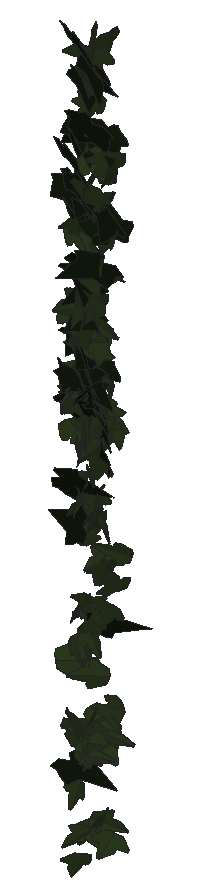
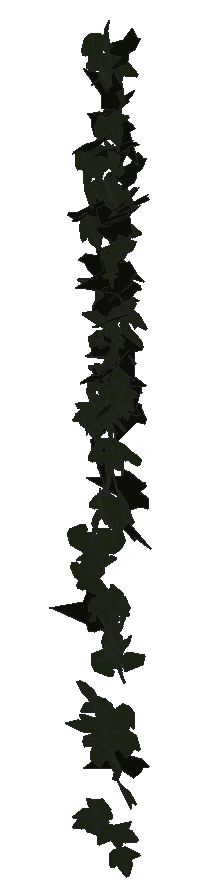
# SketchUp Ruby script. Lengths in inches.
U = 1.inch
M = Sketchup.active_model
def pt(a) = Geom::Point3d.new(a.map { |v| v * U })
def face(e, loops, mat)
  f = e.add_face(loops[0].map { |a| pt(a) })
  loops[1..].each { |l| e.add_face(l.map { |a| pt(a) }).erase! }
  f.material = f.back_material = mat if mat
  f
end
# faces: each face lists its corners as indices into pts; further lists are holes
def faces(e, pts, list, mat = nil) = list.each { |f| face(e, (f[0].is_a?(Array) ? f : [f]).map { |l| l.map { |i| pts[i] } }, mat) }
# xy, xz, yz: faces in a plane at the given z, y or x. An outline is a flat list of corners, or four numbers for a rectangle; further outlines are holes
def ring(l) = l.size == 4 ? [[l[0], l[1]], [l[2], l[1]], [l[2], l[3]], [l[0], l[3]]] : l.each_slice(2).to_a
def flat(e, list, mat, &to3) = list.each { |f| face(e, (f[0].is_a?(Array) ? f : [f]).map { |l| ring(l).map { |u, v| to3.(u, v) } }, mat) }
def xy(e, z, list, mat = nil) = flat(e, list, mat) { |x, y| [x, y, z] }
def xz(e, y, list, mat = nil) = flat(e, list, mat) { |x, z| [x, y, z] }
def yz(e, x, list, mat = nil) = flat(e, list, mat) { |y, z| [x, y, z] }
def lines(e, pts, list) = list.each { |a, b| e.add_line(pt(pts[a]), pt(pts[b])) }
# prism: a flat outline (further loops are holes) pulled along v
def prism(e, loops, v, mat = nil)
  f = face(e, loops, mat); d = Geom::Vector3d.new(v.map { |x| x * U })
  f.pushpull(f.normal.samedirection?(d) ? d.length : -d.length)
end
def box(e, o, s, mat = nil) = prism(e, [[o, [o[0] + s[0], o[1], o[2]], [o[0] + s[0], o[1] + s[1], o[2]], [o[0], o[1] + s[1], o[2]]]], [0, 0, s[2]], mat)
def at(x, y, z, deg = 0) = Geom::Transformation.translation(pt([x, y, z])) * Geom::Transformation.rotation(ORIGIN, Z_AXIS, deg.degrees)
def axes(o, x, y, z) = Geom::Transformation.new([*x, 0, *y, 0, *z, 0, *pt(o).to_a, 1])
def part(name) = M.definitions.add(name)
# library, detail: a bought-in or finely detailed component or shape, given as its bounding box
def library(name, o, s) = part(name).tap { |d| box(d.entities, o, s) }
def detail(e, o, s) = box(e.add_group.entities, o, s)
def put(e, d, t, mat = nil) = e.add_instance(d, t).tap { |i| i.material = mat if mat }
def group(e, t, mat = nil) = e.add_group.tap { |g| g.transformation = t; g.material = mat if mat }.entities
root = M.entities
M.materials.add("1026 AP 7946 SUNNY SIDE UP").color = [254, 231, 186]
M.materials.add("efeu1").color = [18, 25, 13]
M.materials.add("efeu2").color = [43, 57, 29]
c1 = part("ivyleaf_9")
p = [[1.54,2.16,1.25],[1.36,2.04,1.19],[-0.21,0.99,0.68],[-0.71,1.11,0.82],[-0.85,0.86,0.67],[-0.8,0.17,0.21],
  [-0.9,-0.01,0.1],[-0.67,-0.16,-0.02],[-0.08,-0.08,-0.05],[-0.03,-0.6,-0.4],[0.65,-0.88,-0.66],[0.83,-0.6,-0.49],
  [1.29,-0.42,-0.43],[1.8125,-0.07,-0.26],[1.21,0.44,0.15]]
faces(c1.entities,p,[[0,1,2,3,4,5,6,7,8,9,10,11,12,13,14]],"efeu1")
c2 = part("ivyleaf_10")
p = [[0,0.5,-0.03],[-0.0625,2.02,-0.43],[-0.19,2.01,-0.46],[-0.54,1.05,-0.29],[-0.52,0.625,-0.18],[-0.83,0.76,-0.28],
  [-1.16,0.64,-0.33],[-1.15,0.33,-0.24],[-0.77,-0.39,0.02],[-0.3,-0.51,0.16],[0.04,-0.48,0.23],[-0.02,2.01,-0.4375],
  [-0.06,2.01,-0.43],[0.04,-0.49,0.23],[0.67,-0.49,0.14],[1.38,0.36,-0.2],[1.375,0.51,-0.24],[0.81,0.65,-0.19],
  [0.62,0.59,-0.15],[0.6,1.09,-0.28],[0.5,1.23,-0.31]]
faces(c2.entities,p,[[0,1,2,3,4,5,6,7,8,9,10],[11,12,0,13,14,15,16,17,18,19,20]],"efeu2")
put(root,c1,axes([104.4,212.4,264.42],[0.02989,-0.26168,-0.05002],[-0.00858,0.0468,-0.27001],[0.41798,0.01967,-0.00197]),"1026 AP 7946 SUNNY SIDE UP")
put(root,c1,axes([104.31,212.37,265.12],[0.20144,-0.21294,0.07682],[0.04069,-0.07271,-0.25599],[0.35306,0.12988,-0.01432]),"1026 AP 7946 SUNNY SIDE UP")
put(root,c2,axes([104.32,212.5625,259.23],[0.25489,0.03596,0.15428],[0.23922,-0.00544,-0.16856],[-0.03566,0.22049,-0.028]),"1026 AP 7946 SUNNY SIDE UP")
put(root,c1,axes([104.85,212.17,257.49],[-0.16935,-0.01867,-0.23851],[-0.36458,0.02183,0.10948],[0.01886,0.25432,-0.0254]),"1026 AP 7946 SUNNY SIDE UP")
put(root,c2,axes([104.61,212.53,260.5],[0.32823,-0.01925,-0.08265],[-0.12677,-0.00257,-0.21576],[0.02681,0.22358,-0.00828]),"1026 AP 7946 SUNNY SIDE UP")
put(root,c2,axes([104.83,212.23,262.04],[-0.19983,0.01215,0.215],[-0.3172,-0.0709,-0.12276],[0.08582,-0.23378,0.04691]),"1026 AP 7946 SUNNY SIDE UP")
put(root,c2,axes([104.5,212.45,253.1],[-0.29451,-0.02372,-0.08377],[0.13034,-0.01233,-0.19339],[0.02639,-0.20377,0.02024]),"1026 AP 7946 SUNNY SIDE UP")
put(root,c2,axes([104.37,212.42,261.75],[0.28025,-0.04811,0.18082],[0.24774,-0.08293,-0.18843],[0.14407,0.2362,-0.02772]),"1026 AP 7946 SUNNY SIDE UP")
put(root,c1,axes([104.74,212.24,260.06],[0.1133,-0.04955,0.23654],[-0.1924,0.19742,0.08451],[-0.31578,-0.13807,0.03338]),"1026 AP 7946 SUNNY SIDE UP")
put(root,c1,axes([104.5,212.41,265.51],[0.24093,-0.15823,-0.14785],[-0.17433,0.09078,-0.22593],[0.28602,0.18862,-0.01316]),"1026 AP 7946 SUNNY SIDE UP")
put(root,c2,axes([104.59,212.35,260.125],[0.03534,-0.14597,0.17818],[0.046,-0.17132,-0.15314],[0.35389,0.03684,0.00211]),"1026 AP 7946 SUNNY SIDE UP")
put(root,c2,axes([104.6,212.45,257.78],[-0.07078,-0.19746,-0.10932],[0.05848,0.099,-0.20766],[0.34676,-0.057,0.01271]),"1026 AP 7946 SUNNY SIDE UP")
put(root,c2,axes([104.65,212.36,263.78],[-0.11542,-0.23449,-0.01715],[0.00878,0.0143,-0.25304],[0.36939,-0.07361,0.00066]),"1026 AP 7946 SUNNY SIDE UP")
put(root,c1,axes([104.53,212.66,264.17],[-0.11975,-0.19196,0.15357],[0.03496,-0.16214,-0.20286],[0.38162,-0.04539,0.06677]),"1026 AP 7946 SUNNY SIDE UP")
put(root,c2,axes([104.6875,212.45,257.67],[-0.22727,0.15109,-0.03318],[-0.02909,0.02804,0.21548],[0.24145,0.14559,-0.00527]),"1026 AP 7946 SUNNY SIDE UP")
put(root,c1,axes([104.44,212.47,264.52],[0.14828,-0.23824,0.00096],[-0.0061,-0.00399,-0.26393],[0.37458,0.09425,-0.00468]),"1026 AP 7946 SUNNY SIDE UP")
put(root,c2,axes([104.53,212.4,263.51],[0.11016,0.22946,0.07194],[0.04535,0.0628,-0.24662],[-0.37381,0.07524,-0.00872]),"1026 AP 7946 SUNNY SIDE UP")
put(root,c1,axes([104.61,212.23,260],[0.33334,0.0588,-0.11051],[-0.15105,-0.05394,-0.22564],[-0.11984,0.23154,-0.02299]),"1026 AP 7946 SUNNY SIDE UP")
put(root,c2,axes([104.7,212.26,258.9],[0.00661,-0.00651,-0.23275],[-0.03665,0.22472,-0.00581],[0.35345,0.02342,0.00375]),"1026 AP 7946 SUNNY SIDE UP")
put(root,c2,axes([104.65,212.47,252.3125],[0.13679,-0.14464,0.12123],[-0.08114,0.10705,0.17426],[-0.28259,-0.10075,0.00865]),"1026 AP 7946 SUNNY SIDE UP")
put(root,c1,axes([104.76,212.44,261.4],[0.14498,0.12771,-0.19277],[-0.14162,-0.16555,-0.16247],[-0.32788,0.12798,-0.01506]),"1026 AP 7946 SUNNY SIDE UP")
put(root,c2,axes([104.64,212.17,253.39],[-0.25694,0.13165,-0.01009],[-0.00282,-0.01898,-0.21567],[-0.20765,-0.16264,0.01542]),"1026 AP 7946 SUNNY SIDE UP")
put(root,c2,axes([104.73,212.35,260.19],[-0.18599,-0.15209,0.15492],[-0.05259,-0.15753,-0.19106],[0.33314,-0.10978,0.05633]),"1026 AP 7946 SUNNY SIDE UP")
put(root,c2,axes([104.61,212.34,251.87],[0.27254,-0.13581,0.04207],[0.0368,-0.03744,-0.22655],[0.22029,0.17427,-0.01421]),"1026 AP 7946 SUNNY SIDE UP")
put(root,c2,axes([104.71,212.39,250.9],[-0.04074,-0.1,0.1821],[-0.03764,-0.17602,-0.10689],[0.31789,-0.03365,0.01068]),"1026 AP 7946 SUNNY SIDE UP")
put(root,c2,axes([104.82,212.09,262.1],[0.08822,-0.12808,-0.23163],[-0.19621,0.18731,-0.14137],[0.35531,0.13524,-0.02056]),"1026 AP 7946 SUNNY SIDE UP")
put(root,c2,axes([104.71,212.3125,250.41],[-0.13218,-0.17999,0.05105],[-0.01944,-0.04998,-0.20471],[0.29334,-0.08442,0.00944]),"1026 AP 7946 SUNNY SIDE UP")
put(root,c2,axes([104.64,212.59,259.1],[0.2023,0.1578,-0.05612],[-0.03973,-0.05072,-0.20968],[-0.25994,0.13056,-0.01163]),"1026 AP 7946 SUNNY SIDE UP")
put(root,c1,axes([104.34,212.26,258.27],[0.17162,0.03856,-0.22421],[0.27273,0.13589,0.11509],[0.21596,-0.20225,0.03282]),"1026 AP 7946 SUNNY SIDE UP")
put(root,c2,axes([104.73,212.48,266.17],[0.22106,-0.17971,-0.14914],[-0.0654,0.14583,-0.22888],[0.3559,0.13842,0.05058]),"1026 AP 7946 SUNNY SIDE UP")
put(root,c2,axes([104.72,212.44,254.66],[0.16577,-0.18209,-0.04436],[-0.0454,0.0318,-0.21638],[0.29032,0.10895,-0.00851]),"1026 AP 7946 SUNNY SIDE UP")
put(root,c1,axes([104.52,212.35,264.1],[0.20084,-0.20444,-0.05932],[-0.04789,0.0475,-0.24806],[0.33002,0.13131,0.00011]),"1026 AP 7946 SUNNY SIDE UP")
put(root,c2,axes([104.64,212.38,261.36],[-0.03415,-0.13729,-0.19819],[0.11714,0.17855,-0.13945],[0.35163,-0.07281,0.02721]),"1026 AP 7946 SUNNY SIDE UP")
put(root,c2,axes([104.64,212.27,254.9375],[0.02045,0.21136,0.01667],[0.00065,0.01498,-0.21806],[-0.33317,0.013,0.0006]),"1026 AP 7946 SUNNY SIDE UP")
put(root,c2,axes([104.72,212.21,255.74],[0.05952,-0.17736,-0.11889],[0.00236,0.11645,-0.18479],[0.33185,0.03099,0.02264]),"1026 AP 7946 SUNNY SIDE UP")
put(root,c2,axes([104.72,212.56,255.27],[0.05189,-0.21191,0.05899],[0.00316,-0.05882,-0.22117],[0.34564,0.03235,-0.00684]),"1026 AP 7946 SUNNY SIDE UP")
put(root,c2,axes([104.625,212.47,265.23],[0.18103,-0.23237,0.04226],[0.01082,0.05038,0.26587],[-0.37123,-0.11185,0.02836]),"1026 AP 7946 SUNNY SIDE UP")
put(root,c2,axes([104.48,212.13,254.57],[0.09186,-0.06714,-0.2225],[0.30328,0.13064,0.01269],[0.18463,-0.18119,0.08985]),"1026 AP 7946 SUNNY SIDE UP")
put(root,c2,axes([104.77,212.25,260.29],[-0.32411,0.15872,-0.0115],[0.00397,0.023,0.26737],[0.25027,0.20519,-0.01914]),"1026 AP 7946 SUNNY SIDE UP")
put(root,c2,axes([104.77,212.65,266.16],[-0.13137,-0.20015,0.13279],[0.00083,-0.13793,-0.21916],[0.3753,-0.06975,0.04697]),"1026 AP 7946 SUNNY SIDE UP")
put(root,c2,axes([104.63,212.46,258.29],[0.23018,-0.13321,0.11784],[0.12203,-0.08559,-0.20416],[0.24851,0.16541,-0.00889]),"1026 AP 7946 SUNNY SIDE UP")
put(root,c1,axes([104.72,212.36,261.11],[0.20799,-0.09581,-0.19009],[-0.24572,0.09747,-0.16746],[0.21449,0.20456,-0.00751]),"1026 AP 7946 SUNNY SIDE UP")
put(root,c1,axes([104.63,212.58,265.63],[-0.07708,-0.24624,-0.01975],[0.01844,0.01578,-0.25842],[0.38776,-0.0497,0.00836]),"1026 AP 7946 SUNNY SIDE UP")
put(root,c1,axes([104.58,212.625,266.51],[-0.02104,-0.2071,0.15439],[0.05871,-0.15121,-0.21107],[0.39875,0.01134,0.03922]),"1026 AP 7946 SUNNY SIDE UP")
put(root,c2,axes([104.53,212.41,252.93],[-0.12964,-0.0363,-0.1905],[0.29283,0.01369,-0.08833],[0.04318,-0.20182,0.02705]),"1026 AP 7946 SUNNY SIDE UP")
put(root,c1,axes([104.5,212.67,263.93],[-0.03753,-0.05014,0.24504],[0.24353,-0.1877,-0.02582],[0.29517,0.14849,0.05246]),"1026 AP 7946 SUNNY SIDE UP")
put(root,c1,axes([104.62,212.47,262.51],[-0.00964,-0.20211,0.13903],[0.02701,-0.13616,-0.2083],[0.38218,0.00452,0.01823]),"1026 AP 7946 SUNNY SIDE UP")
put(root,c2,axes([104.74,212.38,260.66],[-0.21966,0.20066,-0.01863],[-0.00032,-0.02353,-0.25163],[-0.31697,-0.13904,0.01316]),"1026 AP 7946 SUNNY SIDE UP")
put(root,c1,axes([104.49,212.37,262.78],[0.31408,0.07032,0.15021],[0.23278,0.01278,-0.21579],[-0.10157,0.24674,-0.03007]),"1026 AP 7946 SUNNY SIDE UP")
put(root,c1,axes([104.71,212.55,260.96],[-0.09346,-0.15157,0.20757],[-0.03004,-0.20458,-0.16485],[0.3964,-0.05124,0.03645]),"1026 AP 7946 SUNNY SIDE UP")
put(root,c2,axes([104.77,212.51,255.58],[-0.23717,0.14431,-0.00769],[-0.00694,-0.01657,-0.21459],[-0.22719,-0.15015,0.01459]),"1026 AP 7946 SUNNY SIDE UP")
put(root,c1,axes([104.83,212.59,262.38],[-0.02623,-0.04337,-0.24879],[0.10637,-0.23324,0.03701],[-0.37046,-0.0639,0.02824]),"1026 AP 7946 SUNNY SIDE UP")
put(root,c1,axes([104.53,212.33,267.59],[0.18723,-0.21887,0.12623],[0.08053,-0.11296,-0.25721],[0.38707,0.12937,-0.00754]),"1026 AP 7946 SUNNY SIDE UP")
put(root,c2,axes([104.66,212.25,260.01],[-0.22955,-0.1153,-0.16355],[0.23175,0.06496,-0.18863],[0.20239,-0.20515,0.03049]),"1026 AP 7946 SUNNY SIDE UP")
put(root,c2,axes([104.88,212.49,255.76],[-0.34473,-0.03433,0.04347],[-0.05951,-0.03074,-0.22744],[0.06178,-0.22117,0.02351]),"1026 AP 7946 SUNNY SIDE UP")
put(root,c2,axes([104.85,212.43,267.32],[-0.39172,-0.10153,0.00081],[0.01231,-0.02279,-0.27616],[0.15919,-0.24808,0.02334]),"1026 AP 7946 SUNNY SIDE UP")
put(root,c2,axes([104.84,212.5,257.98],[-0.29732,-0.09767,-0.00009],[0.01236,-0.01623,-0.21855],[0.15308,-0.18839,0.01747]),"1026 AP 7946 SUNNY SIDE UP")
put(root,c2,axes([104.98,212.26,262.22],[-0.32027,-0.04262,0.12058],[-0.1683,-0.05578,-0.21269],[0.1009,-0.22832,0.02799]),"1026 AP 7946 SUNNY SIDE UP")
put(root,c2,axes([105.05,212.38,261.32],[0.21917,-0.05349,-0.22711],[-0.33627,0.05428,-0.15275],[0.11761,0.25485,-0.01351]),"1026 AP 7946 SUNNY SIDE UP")
put(root,c1,axes([104.87,212.52,261.81],[-0.22125,-0.14511,0.15397],[-0.08418,-0.15009,-0.20182],[0.31751,-0.14091,0.05378]),"1026 AP 7946 SUNNY SIDE UP")
put(root,c2,axes([104.75,212.39,257.07],[-0.00794,-0.18001,0.14148],[0.03375,0.13739,0.18577],[-0.3554,0.01707,0.01448]),"1026 AP 7946 SUNNY SIDE UP")
put(root,c1,axes([105.03,212.23,265.94],[0.15446,0.02989,-0.25704],[-0.34671,-0.11861,-0.10469],[-0.19006,0.24066,-0.01791]),"1026 AP 7946 SUNNY SIDE UP")
put(root,c2,axes([104.86,212.27,261.94],[0.10784,-0.19761,-0.12152],[0.00674,0.12302,-0.21104],[0.3609,0.05675,0.04026]),"1026 AP 7946 SUNNY SIDE UP")
put(root,c2,axes([104.58,212.52,266.59],[-0.10393,0.03422,0.2773],[0.37706,-0.12185,0.07596],[0.199,0.24874,0.00089]),"1026 AP 7946 SUNNY SIDE UP")
put(root,c2,axes([104.76,212.61,260.41],[0.36,-0.00909,0.0394],[0.05846,-0.02426,-0.23505],[0.02032,0.23086,-0.02178]),"1026 AP 7946 SUNNY SIDE UP")
put(root,c2,axes([104.71,212.46,250.98],[0.17609,0.13997,0.10842],[0.12299,0.07075,-0.18364],[-0.24554,0.13582,-0.01423]),"1026 AP 7946 SUNNY SIDE UP")
put(root,c2,axes([104.875,212.28,264.52],[-0.41283,0.01817,-0.01666],[0.0224,-0.02856,-0.26981],[-0.03113,-0.2615,0.02676]),"1026 AP 7946 SUNNY SIDE UP")
put(root,c2,axes([104.91,212.36,261.46],[-0.13186,-0.2221,0.01168],[0.00217,-0.01398,-0.24457],[0.34978,-0.08364,0.00592]),"1026 AP 7946 SUNNY SIDE UP")
put(root,c1,axes([104.63,212.17,252.46],[0.02405,-0.05517,-0.2474],[0.17891,0.21465,-0.04214],[0.34312,-0.10806,0.03931]),"1026 AP 7946 SUNNY SIDE UP")
put(root,c2,axes([104.86,212.59,267.28],[0.1006,-0.22583,0.11431],[0.04806,-0.108,-0.24244],[0.39362,0.07091,0.00039]),"1026 AP 7946 SUNNY SIDE UP")
put(root,c2,axes([104.9,212.4,264.68],[0.10437,-0.23867,0.03512],[0.00444,-0.03599,-0.25532],[0.37938,0.06608,-0.00667]),"1026 AP 7946 SUNNY SIDE UP")
put(root,c2,axes([104.98,212.27,259.61],[-0.06129,0.1726,0.12521],[-0.16204,0.09128,-0.16841],[-0.28868,-0.08788,0.06795]),"1026 AP 7946 SUNNY SIDE UP")
put(root,c2,axes([104.98,212.52,259.07],[-0.07554,-0.13893,0.16223],[-0.05847,-0.15418,-0.15196],[0.32593,-0.05986,0.01034]),"1026 AP 7946 SUNNY SIDE UP")
put(root,c2,axes([104.95,212.52,262.14],[-0.11182,-0.21033,0.06343],[-0.01243,-0.06348,-0.22874],[0.3449,-0.07048,0.01232]),"1026 AP 7946 SUNNY SIDE UP")
put(root,c2,axes([104.75,212.36,259.34],[0.03951,-0.03825,0.21367],[0.22445,-0.15098,-0.04733],[0.24459,0.14473,0.00892]),"1026 AP 7946 SUNNY SIDE UP")
put(root,c2,axes([104.86,212.24,255.72],[0.01391,-0.06041,0.2209],[0.00408,0.21495,0.06344],[-0.35078,0.0001,0.00949]),"1026 AP 7946 SUNNY SIDE UP")
put(root,c2,axes([104.6,212.5,260.62],[-0.00732,-0.00319,0.26632],[0.40635,-0.00835,0.00464],[0.01304,0.25844,0.00495]),"1026 AP 7946 SUNNY SIDE UP")
put(root,c1,axes([104.67,212.27,260.625],[-0.04569,-0.12066,-0.23083],[0.27753,0.15202,-0.10735],[0.28696,-0.16623,0.06708]),"1026 AP 7946 SUNNY SIDE UP")
put(root,c2,axes([105.01,212.29,258.36],[0.07914,-0.03897,-0.24952],[-0.07798,0.24031,-0.04909],[0.37744,0.05782,0.04218]),"1026 AP 7946 SUNNY SIDE UP")
put(root,c2,axes([104.85,212.57,254.98],[0.07844,-0.12054,0.16802],[0.12778,-0.14277,-0.13458],[0.29311,0.0945,0.0137]),"1026 AP 7946 SUNNY SIDE UP")
put(root,c2,axes([104.99,212.29,253.3],[0.03353,-0.02533,0.22502],[-0.13341,0.20166,0.03378],[-0.31922,-0.08694,0.00951]),"1026 AP 7946 SUNNY SIDE UP")
put(root,c2,axes([104.97,212.43,263.09],[0.27093,-0.14616,-0.0937],[-0.062,0.09058,-0.22847],[0.26278,0.17206,0.0427]),"1026 AP 7946 SUNNY SIDE UP")
put(root,c2,axes([104.82,212.69,257.84],[0.03105,-0.10683,-0.19045],[0.08922,-0.17572,0.1102],[-0.3228,-0.05884,0.01214]),"1026 AP 7946 SUNNY SIDE UP")
put(root,c1,axes([104.73,212.54,260.15],[0.15425,-0.24341,0.06382],[0.0163,-0.06401,-0.27036],[0.39515,0.09766,-0.01376]),"1026 AP 7946 SUNNY SIDE UP")
put(root,c1,axes([104.625,212.57,266.82],[0.19236,-0.04652,-0.23704],[0.36783,0.0064,0.12699],[-0.02534,-0.26028,0.04391]),"1026 AP 7946 SUNNY SIDE UP")
put(root,c2,axes([104.7,212.41,259.61],[0.14344,-0.11461,-0.21992],[0.28724,-0.11628,0.1445],[-0.24891,-0.20024,0.04001]),"1026 AP 7946 SUNNY SIDE UP")
put(root,c2,axes([104.9,212.3125,253.08],[-0.15989,-0.16288,0.09355],[0.06851,0.0809,0.19822],[-0.28585,0.1105,-0.00482]),"1026 AP 7946 SUNNY SIDE UP")
put(root,c2,axes([104.99,212.59,256.64],[-0.07779,-0.00955,0.21063],[0.03546,-0.20937,-0.00568],[0.31996,0.02088,0.05184]),"1026 AP 7946 SUNNY SIDE UP")
put(root,c1,axes([105.17,212.35,263.02],[0.02146,-0.00599,-0.2537],[-0.17784,-0.21922,-0.00225],[-0.34404,0.11295,-0.01466]),"1026 AP 7946 SUNNY SIDE UP")
put(root,c2,axes([105.0625,212.38,258.83],[-0.3185,0.05766,0.04894],[-0.08038,-0.00817,-0.2159],[-0.08522,-0.20782,0.02075]),"1026 AP 7946 SUNNY SIDE UP")
put(root,c2,axes([105.04,212.55,252.6],[-0.03695,-0.10912,0.18433],[-0.0157,-0.17988,-0.11502],[0.32999,-0.02078,0.01517]),"1026 AP 7946 SUNNY SIDE UP")
put(root,c2,axes([105.16,212.33,254.375],[-0.0006,0.01117,0.2362],[-0.17911,-0.19899,0.00863],[0.31325,-0.11376,0.00539]),"1026 AP 7946 SUNNY SIDE UP")
put(root,c1,axes([105.13,212.21,260.53],[-0.1602,0.21433,-0.11562],[0.06167,-0.10687,-0.24491],[-0.3763,-0.10876,0.00908]),"1026 AP 7946 SUNNY SIDE UP")
put(root,c1,axes([105.14,212.43,259.03],[0.1271,-0.02458,-0.23393],[-0.35077,0.04248,-0.08635],[0.07601,0.23712,-0.00733]),"1026 AP 7946 SUNNY SIDE UP")
put(root,c1,axes([104.93,212.64,260.72],[-0.10323,-0.23277,0.018],[0.00087,-0.01967,-0.2492],[0.3672,-0.06539,0.00565]),"1026 AP 7946 SUNNY SIDE UP")
put(root,c2,axes([105.04,212.34,255.68],[-0.25414,-0.14151,0.00621],[0.00824,-0.01632,-0.22081],[0.22262,-0.16094,0.01525]),"1026 AP 7946 SUNNY SIDE UP")
put(root,c2,axes([104.85,212.4,261.12],[0.27808,0.06775,-0.16129],[0.19024,0.10993,0.18998],[0.1899,-0.20934,0.04587]),"1026 AP 7946 SUNNY SIDE UP")
put(root,c2,axes([104.9375,212.43,252.86],[0.13136,0.18617,0.02538],[0.02803,0.01782,-0.20991],[-0.29374,0.08496,-0.00868]),"1026 AP 7946 SUNNY SIDE UP")
put(root,c2,axes([104.97,212.5,259.99],[-0.23655,-0.13836,-0.06824],[0.11053,0.01907,-0.20786],[0.21379,-0.16295,0.03196]),"1026 AP 7946 SUNNY SIDE UP")
put(root,c2,axes([104.77,212.4,262.56],[0.05915,-0.00136,-0.25255],[0.3349,0.12298,0.03369],[0.19086,-0.21537,0.01915]),"1026 AP 7946 SUNNY SIDE UP")
put(root,c2,axes([104.92,212.31,257.75],[0.32738,-0.08053,0.09138],[0.11941,-0.05001,-0.22953],[0.14639,0.2209,-0.01712]),"1026 AP 7946 SUNNY SIDE UP")
put(root,c2,axes([105.19,212.36,259.9],[-0.13969,0.15553,0.12424],[-0.22687,0.03734,-0.16005],[-0.20922,-0.14433,0.0906]),"1026 AP 7946 SUNNY SIDE UP")
put(root,c2,axes([105.15,212.43,252.82],[0.2389,0.08094,-0.15178],[-0.18466,-0.09184,-0.17673],[-0.19001,0.19103,-0.01907]),"1026 AP 7946 SUNNY SIDE UP")
put(root,c2,axes([105.1,212.34,257.82],[0.03859,-0.24701,0.01666],[-0.0007,-0.0177,-0.25581],[0.38938,0.02445,-0.00211]),"1026 AP 7946 SUNNY SIDE UP")
put(root,c2,axes([104.9375,212.43,267.76],[0.12139,-0.14076,0.22254],[0.21559,-0.16953,-0.16467],[0.34458,0.15566,0.02463]),"1026 AP 7946 SUNNY SIDE UP")
put(root,c2,axes([105.12,212.45,251.36],[-0.00208,-0.20628,-0.0474],[-0.00066,0.04484,-0.21225],[0.33193,-0.00121,-0.00072]),"1026 AP 7946 SUNNY SIDE UP")
put(root,c2,axes([104.95,212.34,265.17],[0.17549,0.1953,0.11962],[0.11292,0.09111,-0.23067],[-0.33801,0.13184,-0.01496]),"1026 AP 7946 SUNNY SIDE UP")
put(root,c2,axes([104.875,212.34,255.23],[0.23116,-0.02841,0.19076],[0.27052,-0.07317,-0.15258],[0.11718,0.22496,-0.02406]),"1026 AP 7946 SUNNY SIDE UP")
put(root,c1,axes([104.95,212.39,267.08],[0.04257,-0.24414,0.08882],[-0.00145,-0.08817,-0.25336],[0.40785,0.02517,-0.01017]),"1026 AP 7946 SUNNY SIDE UP")
put(root,c2,axes([104.95,212.61,256.66],[0.01775,-0.02816,-0.20827],[0.13997,-0.18135,0.03011],[-0.28856,-0.0897,0.00179]),"1026 AP 7946 SUNNY SIDE UP")
put(root,c2,axes([104.97,212.35,257.98],[0.20416,-0.12181,0.15689],[0.16692,-0.11032,-0.18395],[0.25824,0.16761,-0.00513]),"1026 AP 7946 SUNNY SIDE UP")
put(root,c2,axes([104.86,212.22,252.71],[-0.01931,-0.03101,-0.2084],[0.31844,0.02616,-0.01666],[0.04447,-0.2008,0.02879]),"1026 AP 7946 SUNNY SIDE UP")
put(root,c2,axes([105.15,212.4375,257.51],[-0.16445,0.18306,0.10958],[-0.096,0.08631,-0.21648],[-0.31791,-0.12076,0.00869]),"1026 AP 7946 SUNNY SIDE UP")
put(root,c2,axes([105.15,212.26,256.53],[0.01212,0.02693,0.21356],[-0.11489,0.19454,-0.02211],[-0.30771,-0.07158,0.01667]),"1026 AP 7946 SUNNY SIDE UP")
put(root,c2,axes([105.15,212.5625,267.71],[-0.08552,-0.24695,-0.03696],[0.0262,0.0316,-0.26014],[0.3912,-0.05611,0.00934]),"1026 AP 7946 SUNNY SIDE UP")
put(root,c2,axes([105.11,212.38,259.73],[-0.35033,-0.05966,-0.03958],[0.06619,-0.01058,-0.23671],[0.08947,-0.22578,0.02014]),"1026 AP 7946 SUNNY SIDE UP")
put(root,c2,axes([104.84,212.41,261.7],[0.03452,0.01456,0.25051],[0.38292,-0.00125,-0.02259],[-0.0001,0.24407,-0.01363]),"1026 AP 7946 SUNNY SIDE UP")
put(root,c2,axes([105.03,212.3,252.9375],[-0.05783,-0.08135,-0.2001],[0.19237,0.15166,-0.08862],[0.26869,-0.12609,0.02039]),"1026 AP 7946 SUNNY SIDE UP")
put(root,c2,axes([105.09,212.21,255.58],[-0.09902,-0.12656,-0.16786],[0.12962,0.13992,-0.1446],[0.29641,-0.10347,0.00716]),"1026 AP 7946 SUNNY SIDE UP")
put(root,c1,axes([105.05,212.68,265.65],[-0.03828,-0.25117,-0.00801],[-0.00217,0.00651,-0.25992],[0.39505,-0.0243,-0.0022]),"1026 AP 7946 SUNNY SIDE UP")
put(root,c2,axes([105.16,212.52,256.8125],[0.12689,0.1891,-0.06642],[-0.02665,-0.06396,-0.21198],[-0.31357,0.08196,-0.00886]),"1026 AP 7946 SUNNY SIDE UP")
put(root,c2,axes([105.22,212.15,257.8],[-0.00572,-0.1716,-0.12814],[0.02792,0.12274,-0.17565],[0.33118,-0.01331,0.0126]),"1026 AP 7946 SUNNY SIDE UP")
put(root,c2,axes([105.03,212.44,251.25],[0.07662,0.05066,0.20326],[0.19146,0.15503,-0.07118],[-0.25624,0.13098,0.00759]),"1026 AP 7946 SUNNY SIDE UP")
put(root,c2,axes([104.99,212.42,253.52],[0.17507,0.06087,0.17055],[0.24305,0.05981,-0.12966],[-0.13257,0.19004,-0.01249]),"1026 AP 7946 SUNNY SIDE UP")
put(root,c2,axes([105.27,212.375,264.43],[-0.02126,-0.2317,0.09399],[-0.0052,-0.09251,-0.23964],[0.39228,-0.01379,0.00192]),"1026 AP 7946 SUNNY SIDE UP")
put(root,c2,axes([105.08,212.55,259.82],[-0.24639,-0.02283,-0.15364],[0.23703,-0.02247,-0.1599],[0.00139,-0.21506,0.03173]),"1026 AP 7946 SUNNY SIDE UP")
put(root,c2,axes([105.31,212.48,265.24],[-0.16941,-0.23126,0.0783],[-0.01548,-0.08033,-0.26214],[0.38311,-0.10551,0.02403]),"1026 AP 7946 SUNNY SIDE UP")
put(root,c2,axes([105.27,212.59,259.6875],[-0.12087,0.16346,-0.12523],[-0.06691,-0.14082,-0.16691],[-0.31414,-0.0329,0.08374]),"1026 AP 7946 SUNNY SIDE UP")
put(root,c2,axes([105.34,212.54,259.53],[0.28627,-0.12421,-0.09948],[-0.14023,0.03889,-0.22618],[0.20298,0.20205,-0.01595]),"1026 AP 7946 SUNNY SIDE UP")
put(root,c1,axes([105.05,212.45,259.72],[0.01062,-0.03822,-0.25039],[0.36885,-0.07164,0.01792],[-0.11558,-0.23212,0.03417]),"1026 AP 7946 SUNNY SIDE UP")
put(root,c2,axes([105.33,212.47,263.71],[-0.05606,-0.23677,0.06363],[-0.01025,-0.06284,-0.24702],[0.38516,-0.03613,0.00269]),"1026 AP 7946 SUNNY SIDE UP")
put(root,c2,axes([105.18,212.61,260.23],[0.09375,-0.09167,0.20294],[0.16313,-0.16809,-0.11361],[0.30103,0.11963,-0.00163]),"1026 AP 7946 SUNNY SIDE UP")
put(root,c2,axes([105.31,212.46,250.96],[0.23669,0.11093,-0.08863],[-0.09232,-0.06584,-0.19227],[-0.20117,0.16073,-0.01605]),"1026 AP 7946 SUNNY SIDE UP")
put(root,c1,axes([105.43,212.32,263.74],[-0.34923,-0.11549,0.09949],[0.12152,0.06159,0.25761],[-0.20392,0.23449,-0.01687]),"1026 AP 7946 SUNNY SIDE UP")
put(root,c2,axes([105.4,212.27,255.94],[-0.31785,0.01737,0.05255],[-0.08233,-0.01811,-0.2079],[-0.01941,-0.20767,0.02129]),"1026 AP 7946 SUNNY SIDE UP")
put(root,c2,axes([105.35,212.26,256.8],[-0.09909,-0.21495,0.00384],[0.00436,-0.00597,-0.23075],[0.33805,-0.06293,0.0041]),"1026 AP 7946 SUNNY SIDE UP")
put(root,c2,axes([105.55,212.54,256.97],[-0.06961,0.00962,-0.20891],[-0.31202,-0.04615,0.04209],[-0.06783,0.20242,0.02077]),"1026 AP 7946 SUNNY SIDE UP")
put(root,c2,axes([105.1,212.52,253.11],[-0.09887,-0.03918,-0.2028],[0.31462,0.00097,-0.06611],[0.02025,-0.20644,0.03692]),"1026 AP 7946 SUNNY SIDE UP")
put(root,c2,axes([105.46,212.46,253.78],[0.19469,-0.11607,-0.12696],[-0.16514,0.06605,-0.17333],[0.20782,0.16122,-0.0188]),"1026 AP 7946 SUNNY SIDE UP")
put(root,c2,axes([105.37,212.44,265.06],[0.02436,-0.23041,-0.13725],[0.01428,0.13253,-0.23658],[0.41723,0.00892,0.01611]),"1026 AP 7946 SUNNY SIDE UP")
put(root,c2,axes([105.375,212.49,256.22],[-0.15393,-0.18847,-0.08918],[-0.07172,-0.0726,0.21827],[-0.31742,0.1078,-0.00607]),"1026 AP 7946 SUNNY SIDE UP")
put(root,c2,axes([105.375,212.39,263.74],[0.23641,-0.20563,-0.01791],[-0.0255,0.00822,-0.26224],[0.32334,0.151,-0.00758]),"1026 AP 7946 SUNNY SIDE UP")
put(root,c1,axes([105.07,212.375,255.42],[0.18923,0.04165,0.21772],[0.3305,0.029,-0.12916],[-0.0724,0.24126,-0.02059]),"1026 AP 7946 SUNNY SIDE UP")
put(root,c1,axes([105.29,212.44,264.05],[-0.08615,-0.20724,0.15273],[-0.00112,-0.1527,-0.21933],[0.40173,-0.04487,0.03214]),"1026 AP 7946 SUNNY SIDE UP")
